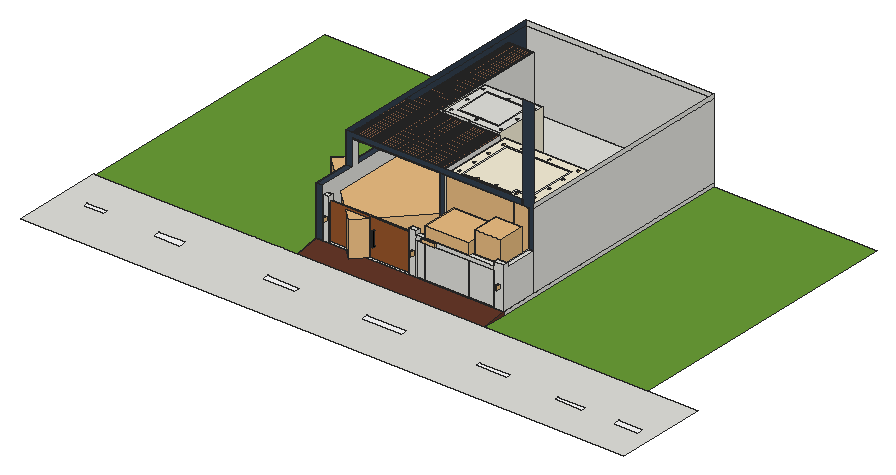
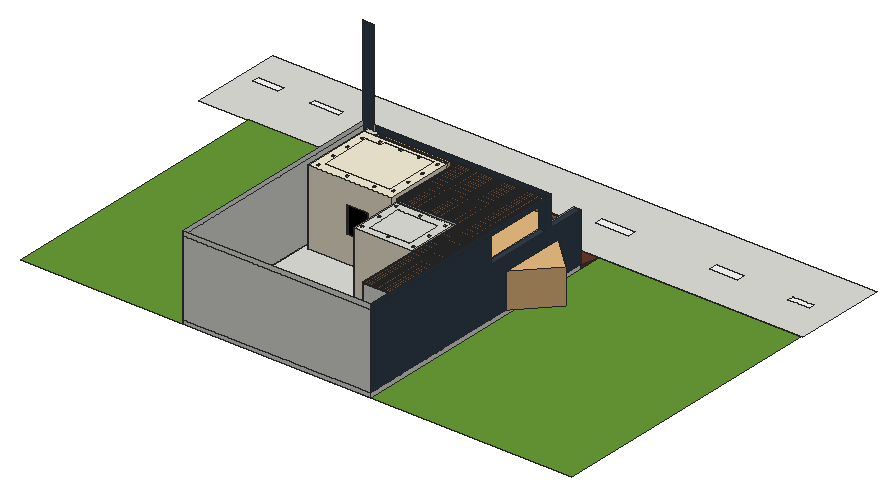
# SketchUp Ruby script. Lengths in inches.
U = 1.inch
M = Sketchup.active_model
def pt(a) = Geom::Point3d.new(a.map { |v| v * U })
def face(e, loops, mat)
  f = e.add_face(loops[0].map { |a| pt(a) })
  loops[1..].each { |l| e.add_face(l.map { |a| pt(a) }).erase! }
  f.material = f.back_material = mat if mat
  f
end
# faces: each face lists its corners as indices into pts; further lists are holes
def faces(e, pts, list, mat = nil) = list.each { |f| face(e, (f[0].is_a?(Array) ? f : [f]).map { |l| l.map { |i| pts[i] } }, mat) }
# xy, xz, yz: faces in a plane at the given z, y or x. An outline is a flat list of corners, or four numbers for a rectangle; further outlines are holes
def ring(l) = l.size == 4 ? [[l[0], l[1]], [l[2], l[1]], [l[2], l[3]], [l[0], l[3]]] : l.each_slice(2).to_a
def flat(e, list, mat, &to3) = list.each { |f| face(e, (f[0].is_a?(Array) ? f : [f]).map { |l| ring(l).map { |u, v| to3.(u, v) } }, mat) }
def xy(e, z, list, mat = nil) = flat(e, list, mat) { |x, y| [x, y, z] }
def xz(e, y, list, mat = nil) = flat(e, list, mat) { |x, z| [x, y, z] }
def yz(e, x, list, mat = nil) = flat(e, list, mat) { |y, z| [x, y, z] }
def lines(e, pts, list) = list.each { |a, b| e.add_line(pt(pts[a]), pt(pts[b])) }
# prism: a flat outline (further loops are holes) pulled along v
def prism(e, loops, v, mat = nil)
  f = face(e, loops, mat); d = Geom::Vector3d.new(v.map { |x| x * U })
  f.pushpull(f.normal.samedirection?(d) ? d.length : -d.length)
end
def box(e, o, s, mat = nil) = prism(e, [[o, [o[0] + s[0], o[1], o[2]], [o[0] + s[0], o[1] + s[1], o[2]], [o[0], o[1] + s[1], o[2]]]], [0, 0, s[2]], mat)
def at(x, y, z, deg = 0) = Geom::Transformation.translation(pt([x, y, z])) * Geom::Transformation.rotation(ORIGIN, Z_AXIS, deg.degrees)
def axes(o, x, y, z) = Geom::Transformation.new([*x, 0, *y, 0, *z, 0, *pt(o).to_a, 1])
def part(name) = M.definitions.add(name)
# library, detail: a bought-in or finely detailed component or shape, given as its bounding box
def library(name, o, s) = part(name).tap { |d| box(d.entities, o, s) }
def detail(e, o, s) = box(e.add_group.entities, o, s)
def put(e, d, t, mat = nil) = e.add_instance(d, t).tap { |i| i.material = mat if mat }
def group(e, t, mat = nil) = e.add_group.tap { |g| g.transformation = t; g.material = mat if mat }.entities
root = M.entities
M.materials.add("0400 AP 7301 PLUTO").color = [50, 63, 78]
M.materials.add("0897 AP 7835 CREAM CARESS").color = [247, 240, 216]
M.materials.add("Ceragres-Topcer-Brick-red-mat-6-4K").color = [99, 54, 40]
M.materials.add("Color_2").color = [255, 255, 255]
M.materials.add("Glass_Window_Neutral").color = [0, 0, 0]
M.materials["Glass_Window_Neutral"].alpha = 0.125
M.materials.add("Material60").color = [234, 198, 157]
M.materials.add("[Color M09]").color = [0, 0, 0]
M.materials.add("[Color M09]1").color = [0, 0, 0]
M.materials.add("[Grass Dark Green]").color = [106, 157, 55]
M.materials.add("[Wood Cherry Original]").color = [152, 86, 42]
M.materials.add("[Wood Veneer 02]").color = [190, 128, 91]
M.materials.add("ground1").color = [30, 21, 16]
M.materials.add("lz-doorbrown").color = [51, 28, 20]
M.materials.add("polished steel").color = [183, 187, 190]
M.materials.add("steel").color = [179, 179, 179]
c1 = part("Untitled")
xy(c1.entities,0,[[[158.81,26.5625,306.06,993.3125],[226.57,518.17,239.57,583.92],[225.28,357.51,237.28,411.51],[222.61,182.28,236.36,226.53],[239.71,931.55,251.46,972.3],[233.64,703.93,242.14,755.18],[240.05,835.03,248.8,880.53],[222.04,66.5,231.29,100.5]]])
xy(c1.entities,0,[[222.04,66.5,231.29,100.5],[222.61,182.28,236.36,226.53],[225.28,357.51,237.28,411.51],[226.57,518.17,239.57,583.92],[233.64,703.93,242.14,755.18],
  [240.05,835.03,248.8,880.53],[239.71,931.55,251.46,972.3]],"Color_2")
c2 = library("Senza",[-37.85,-41.61,-2.42],[41.39,41.83,53.67])
c3 = library("Cay chuoi",[-26.05,-21.66,0],[63.57,52.43,69.02])
c4 = library("шторы раздвинутые\#1",[23.6875,-79.1875,1.01],[68.3125,79.67,5.17])
c5 = library("door by lz",[5.91,-4.92,0],[35.43,6.61,78.74])
c6 = library("Спалня Венид",[0.07,-0.07,0],[84.71,86.8,39])
c7 = library("RANGE ROVER",[-63.71,-35.21,42.76],[182.88,182.88,64.08])
c8 = part("Bilal architect uae abu dhabi ")
put(c8.entities,c7,axes([104.22,-10.75,-48.75],[0.98727,0.57,0],[-0.57,0.98727,0],[0,0,1.14]),"Material60")
c9 = part("faewg")
xy(c9.entities,0,[[0,-3,2,0]])
xy(c9.entities,1,[[0,-2,2,0]])
xy(c9.entities,23,[[0,-2,2,0]])
xy(c9.entities,24,[[0,-3,2,0]])
xz(c9.entities,-3,[[0,0,2,24]],"polished steel")
xz(c9.entities,-2,[[0,1,2,23]])
xz(c9.entities,0,[[0,0,2,1],[0,23,2,24]])
yz(c9.entities,0,[[-3,0,-3,24,0,24,0,23,-2,23,-2,1,0,1,0,0]])
yz(c9.entities,2,[[-3,0,0,0,0,1,-2,1,-2,23,0,23,0,24,-3,24]])
c10 = part("reg")
xy(c10.entities,0,[[-8.95,3,59.93,5]],"[Wood Veneer 02]")
xy(c10.entities,18,[[51.93,0,53.93,3]],"[Wood Veneer 02]")
xy(c10.entities,19,[[51.93,1,53.93,3]],"[Color M09]")
xy(c10.entities,41,[[51.93,1,53.93,3]],"[Color M09]")
xy(c10.entities,42,[[51.93,0,53.93,3]],"[Color M09]")
xy(c10.entities,61,[[-8.95,3,59.93,5]],"[Wood Veneer 02]")
xz(c10.entities,0,[[51.93,18,53.93,42]],"[Color M09]")
xz(c10.entities,1,[[51.93,19,53.93,41]],"[Color M09]")
xz(c10.entities,3,[[[-8.95,0,59.93,61],[51.93,41,53.93,42],[51.93,18,53.93,19]]],"[Wood Cherry Original]")
xz(c10.entities,3,[[51.93,18,53.93,19],[51.93,41,53.93,42]],"[Wood Veneer 02]")
xz(c10.entities,5,[[-8.95,0,59.93,61]],"[Wood Veneer 02]")
yz(c10.entities,-8.95,[[3,0,5,61]],"[Wood Veneer 02]")
yz(c10.entities,51.93,[[0,18,0,42,3,42,3,41,1,41,1,19,3,19,3,18]],"[Color M09]")
yz(c10.entities,53.93,[[0,18,3,18,3,19,1,19,1,41,3,41,3,42,0,42]],"[Color M09]")
yz(c10.entities,59.93,[[3,0,5,61]],"[Wood Veneer 02]")
put(c10.entities,c9,axes([51.93,5.4375,42],[1,0,0],[0,-1,0],[0,0,-1]),"steel")
c11 = part("gbsrtn")
put(c11.entities,c10,at(402.95,-3,0))
put(c11.entities,c10,axes([522.82,-3,0],[-1,0,0],[0,1,0],[0,0,1]),"[Wood Veneer 02]")
c12 = library("Sliding windows",[297.42,-0.89,0.35],[194.88,8.85,122.84])
c13 = library("Group23\#1",[-12,-48,0],[24,96,0.39])
c14 = library("Wall Light 02",[0,0,0],[3.15,6.76,4.53])
c15 = library("JOHN_K",[0.08,0,0],[23.74,5.375,2])
c16 = part("Window")
xy(c16.entities,31.72,[[-0.78,88.6,2.72,128.1]])
xy(c16.entities,34.95,[[0.84,91.53,1.05,97.58],[1.05,91.53,1.42,106.59],[1.42,91.53,2.72,106.59],[0.84,97.58,1.05,98.18],[0.84,98.18,1.05,106.59]])
xy(c16.entities,34.95,[[-0.78,91.53,0.84,106.59]],"[Wood Cherry Original]")
xy(c16.entities,35.27,[[1.05,110.09,2.72,125.14]])
xy(c16.entities,35.27,[[-0.78,110.09,0.97,125.14]],"[Wood Cherry Original]")
xy(c16.entities,58.35,[[2.72,108.74,3.8,109.74]])
xy(c16.entities,77.8125,[[0.97,110.09,1.05,125.14]])
xy(c16.entities,77.8125,[[-0.78,110.09,2.72,125.14]],"[Wood Cherry Original]")
xy(c16.entities,77.93,[[1.05,91.53,1.42,106.59],[1.42,91.53,2.72,106.59]])
xy(c16.entities,77.93,[[-0.78,91.53,0.84,106.59]],"[Wood Cherry Original]")
xy(c16.entities,80.72,[[-0.78,88.6,2.72,128.1]])
xz(c16.entities,88.6,[[-0.78,31.72,2.72,80.72]])
xz(c16.entities,91.53,[[1.05,34.95,1.42,77.93],[1.42,34.95,2.72,77.93]])
xz(c16.entities,91.53,[[-0.78,34.95,0.84,77.93]],"[Wood Cherry Original]")
xz(c16.entities,106.59,[[0.84,34.95,1.05,77.93],[0.84,34.95,2.72,77.93]])
xz(c16.entities,106.59,[[-0.78,34.95,0.84,77.93]],"[Wood Cherry Original]")
xz(c16.entities,108.74,[[3.8,54.35,4.22,54.6,4.22,59.47,2.72,59.97,2.72,58.35,3.8,58.35]])
xz(c16.entities,109.74,[[3.8,54.35,3.8,58.35,2.72,58.35,2.72,59.97,4.22,59.47,4.22,54.6]])
xz(c16.entities,110.09,[[1.05,35.27,2.72,77.8125]])
xz(c16.entities,110.09,[[-0.78,35.27,0.97,77.8125]],"[Wood Cherry Original]")
xz(c16.entities,125.14,[[0.97,35.27,1.05,80.72],[1.05,35.27,2.72,77.8125]])
xz(c16.entities,125.14,[[-0.78,35.27,0.97,77.8125]],"[Wood Cherry Original]")
xz(c16.entities,128.1,[[-0.78,31.72,2.72,80.72]])
yz(c16.entities,-0.78,[[[88.6,31.72,128.1,80.72],[91.53,34.95,106.59,77.93],[110.09,35.27,125.14,77.8125]]],"[Wood Cherry Original]")
yz(c16.entities,1.05,[[91.53,34.95,106.59,77.93],[110.09,35.27,125.14,77.8125]],"Glass_Window_Neutral")
yz(c16.entities,1.42,[[91.53,34.95,106.59,77.93]])
yz(c16.entities,2.72,[[[88.6,31.72,108.35,80.72],[91.53,34.95,106.59,77.93]],[[108.35,31.72,128.1,80.72],[110.09,35.27,125.14,77.8125],[108.74,58.35,109.74,59.97]]])
yz(c16.entities,3.8,[[108.74,54.35,109.74,58.35]])
yz(c16.entities,4.22,[[108.74,54.6,109.74,59.47]])
p = [[4.22,108.74,54.6],[3.8,108.74,54.35],[3.8,109.74,54.35],[4.22,109.74,54.6],[2.72,109.74,59.97],[2.72,108.74,59.97],
  [4.22,108.74,59.47],[4.22,109.74,59.47],[-0.78,86.4,89.94],[-0.78,86.44,89.94],[15.22,130.69,89.94],[15.22,130.65,89.94],
  [-0.78,86.44,28.19],[-0.78,86.4,28.19],[7.72,130.69,89.94],[7.72,130.65,89.94]]
faces(c16.entities,p,[[0,1,2,3],[4,5,6,7]])
lines(c16.entities,p,[[8,9],[10,11],[12,13],[14,15]])
c17 = part("Group\#7")
xy(c17.entities,0,[[1.02,0,0.76,0.03,0.51,0.14,0.3,0.3,0.14,0.51,0.03,0.76,0,1.02,0.03,1.28,0.14,1.53,0.3,1.74,0.51,1.9,0.76,2.01,1.02,2.04,1.28,2.01,1.53,1.9,1.74,1.74,1.9,1.53,2.01,1.28,2.04,1.02,2.01,0.76,1.9,0.51,1.74,0.3,1.53,0.14,1.28,0.03]])
c18 = part("Group\#9")
detail(c18.entities,[3.14,3.14,12.38],[2.62,2.62,0.48])
put(c18.entities,c17,at(3.43,3.43,12.51))
c19 = part("Group450\#1")
box(c19.entities,[-75,-146,0],[1,110,0.375])
c20 = part("Group451\#1")
box(c20.entities,[-73.8125,-146,0],[1,110,0.375])
c21 = part("Group452\#1")
box(c21.entities,[-72.625,-146,0],[1,110,0.375])
c22 = part("Group453\#1")
box(c22.entities,[-71.4375,-146,0],[1,110,0.375])
c23 = part("Group454\#1")
box(c23.entities,[-70.25,-146,0],[1,110,0.375])
c24 = part("Group455\#1")
box(c24.entities,[-69.0625,-146,0],[1,110,0.375])
c25 = part("Group456\#1")
box(c25.entities,[-67.875,-146,0],[1,110,0.375])
c26 = part("Group457\#1")
box(c26.entities,[-66.6875,-146,0],[1,110,0.375])
c27 = part("Group458\#1")
xy(c27.entities,0,[[-65,-156,-65,-146,-65.5,-146,-65.5,-36,-65,-36,-65,156,-64.5,156,-64.5,-156]])
xy(c27.entities,0.375,[[-65,-156,-64.5,-156,-64.5,156,-65,156,-65,-36,-65.5,-36,-65.5,-146,-65,-146]])
yz(c27.entities,-65.5,[[-146,0,-36,0.375]])
yz(c27.entities,-64.5,[[-156,0,156,0.375]])
c28 = part("Group459\#1")
box(c28.entities,[-64.3125,-156,0],[1,312,0.375])
c29 = part("Group460\#1")
box(c29.entities,[-63.125,-156,0],[1,312,0.375])
c30 = part("Group461\#1")
box(c30.entities,[-61.9375,-156,0],[1,312,0.375])
c31 = part("Group462\#1")
box(c31.entities,[-60.75,-156,0],[1,312,0.375])
c32 = part("Group463\#1")
box(c32.entities,[-59.5625,-156,0],[1,312,0.375])
c33 = part("Group464\#1")
box(c33.entities,[-58.375,-156,0],[1,312,0.375])
c34 = part("Group465\#1")
box(c34.entities,[-57.1875,-156,0],[1,312,0.375])
c35 = part("Group466\#1")
box(c35.entities,[-56,-156,0],[1,312,0.375])
c36 = part("Group467\#1")
box(c36.entities,[-54.8125,-156,0],[1,312,0.375])
c37 = part("Group468\#1")
box(c37.entities,[-53.625,-156,0],[1,312,0.375])
c38 = part("Group469\#1")
box(c38.entities,[-52.4375,-156,0],[1,312,0.375])
c39 = part("Group470\#1")
box(c39.entities,[-51.25,-156,0],[1,312,0.375])
c40 = part("Group471\#1")
box(c40.entities,[-50.0625,-156,0],[1,312,0.375])
c41 = part("Group472\#1")
box(c41.entities,[-48.875,-156,0],[1,312,0.375])
c42 = part("Group473\#1")
box(c42.entities,[-47.6875,-156,0],[1,312,0.375])
c43 = part("Group474\#1")
box(c43.entities,[-46.5,-156,0],[1,312,0.375])
c44 = part("Group475\#1")
box(c44.entities,[-45.3125,-156,0],[1,312,0.375])
c45 = part("Group476\#1")
box(c45.entities,[-44.125,-156,0],[1,312,0.375])
c46 = part("Group477\#1")
box(c46.entities,[-42.9375,-156,0],[1,312,0.375])
c47 = part("Group478\#1")
box(c47.entities,[-41.75,-156,0],[1,312,0.375])
c48 = part("Group479\#1")
box(c48.entities,[-40.5625,-156,0],[1,312,0.375])
c49 = part("Group480\#1")
box(c49.entities,[-39.375,-156,0],[1,312,0.375])
c50 = part("Group481\#1")
box(c50.entities,[-38.1875,-156,0],[1,312,0.375])
c51 = part("Group482\#1")
box(c51.entities,[-37,-156,0],[1,312,0.375])
c52 = part("Group483\#1")
box(c52.entities,[-35.8125,-156,0],[1,312,0.375])
c53 = part("Group484\#1")
box(c53.entities,[-34.625,-156,0],[1,312,0.375])
c54 = part("Group485\#1")
box(c54.entities,[-33.4375,-156,0],[1,312,0.375])
c55 = part("Group486\#1")
box(c55.entities,[-32.25,-156,0],[1,312,0.375])
c56 = part("Group487\#1")
box(c56.entities,[-31.0625,-156,0],[1,312,0.375])
c57 = part("Group488\#1")
box(c57.entities,[-29.875,-156,0],[1,312,0.375])
c58 = part("Group489\#1")
box(c58.entities,[-28.6875,-156,0],[1,312,0.375])
c59 = part("Group490\#1")
box(c59.entities,[-27.5,-156,0],[1,312,0.375])
c60 = part("Group491\#1")
box(c60.entities,[-26.3125,-156,0],[1,312,0.375])
c61 = part("Group492\#1")
xy(c61.entities,0,[[-25.125,-156,-25.125,156,-24.3125,156,-24.3125,-36,-24.125,-36,-24.125,-156]])
xy(c61.entities,0.375,[[-25.125,-156,-24.125,-156,-24.125,-36,-24.3125,-36,-24.3125,156,-25.125,156]])
xz(c61.entities,-156,[[-25.125,0,-24.125,0.375]])
yz(c61.entities,-25.125,[[-156,0,156,0.375]])
yz(c61.entities,-24.125,[[-156,0,-36,0.375]])
c62 = part("Group493\#1")
box(c62.entities,[-23.9375,-156,0],[1,120,0.375])
c63 = part("Group494\#1")
box(c63.entities,[-22.75,-156,0],[1,120,0.375])
c64 = part("Group495\#1")
box(c64.entities,[-21.5625,-156,0],[1,120,0.375])
c65 = part("Group496\#1")
box(c65.entities,[-20.375,-156,0],[1,120,0.375])
c66 = part("Group497\#1")
box(c66.entities,[-19.1875,-156,0],[1,120,0.375])
c67 = part("Group498\#1")
box(c67.entities,[-18,-156,0],[1,120,0.375])
c68 = part("Group499\#1")
box(c68.entities,[-16.8125,-156,0],[1,120,0.375])
c69 = part("Group500\#1")
box(c69.entities,[-15.625,-156,0],[1,120,0.375])
c70 = part("Group501\#1")
box(c70.entities,[-14.4375,-156,0],[1,120,0.375])
c71 = part("Group502\#1")
box(c71.entities,[-13.25,-156,0],[1,120,0.375])
c72 = part("Group503\#1")
box(c72.entities,[-12.0625,-156,0],[1,120,0.375])
c73 = part("Group504\#1")
box(c73.entities,[-10.875,-156,0],[1,120,0.375])
c74 = part("Group505\#1")
box(c74.entities,[-9.6875,-156,0],[1,120,0.375])
c75 = part("Group506\#1")
box(c75.entities,[-8.5,-156,0],[1,120,0.375])
c76 = part("Group507\#1")
box(c76.entities,[-7.3125,-156,0],[1,120,0.375])
c77 = part("Group508\#1")
box(c77.entities,[-6.125,-156,0],[1,120,0.375])
c78 = part("Group509\#1")
box(c78.entities,[-4.9375,-156,0],[1,120,0.375])
c79 = part("Group510\#1")
box(c79.entities,[-3.75,-156,0],[1,120,0.375])
c80 = part("Group511\#1")
box(c80.entities,[-2.5625,-156,0],[1,120,0.375])
c81 = part("Group512\#1")
box(c81.entities,[-1.375,-156,0],[1,120,0.375])
c82 = part("Group513\#1")
box(c82.entities,[-0.1875,-156,0],[1,120,0.375])
c83 = part("Group514\#1")
box(c83.entities,[1,-156,0],[1,120,0.375])
c84 = part("Group515\#1")
box(c84.entities,[2.1875,-156,0],[1,120,0.375])
c85 = part("Group516\#1")
box(c85.entities,[3.375,-156,0],[1,120,0.375])
c86 = part("Group517\#1")
box(c86.entities,[4.5625,-156,0],[1,120,0.375])
c87 = part("Group518\#1")
box(c87.entities,[5.75,-156,0],[1,120,0.375])
c88 = part("Group519\#1")
box(c88.entities,[6.9375,-156,0],[1,120,0.375])
c89 = part("Group520\#1")
box(c89.entities,[8.125,-156,0],[1,120,0.375])
c90 = part("Group521\#1")
box(c90.entities,[9.3125,-156,0],[1,120,0.375])
c91 = part("Group522\#1")
box(c91.entities,[10.5,-156,0],[1,120,0.375])
c92 = part("Group523\#1")
box(c92.entities,[11.6875,-156,0],[1,120,0.375])
c93 = part("Group524\#1")
box(c93.entities,[12.875,-156,0],[1,120,0.375])
c94 = part("Group525\#1")
box(c94.entities,[14.0625,-156,0],[1,120,0.375])
c95 = part("Group526\#1")
box(c95.entities,[15.25,-156,0],[1,120,0.375])
c96 = part("Group527\#1")
box(c96.entities,[16.4375,-156,0],[1,120,0.375])
c97 = part("Group528\#1")
box(c97.entities,[17.625,-156,0],[1,120,0.375])
c98 = part("Group529\#1")
box(c98.entities,[18.8125,-156,0],[1,120,0.375])
c99 = part("Group530\#1")
box(c99.entities,[20,-156,0],[1,120,0.375])
c100 = part("Group531\#1")
box(c100.entities,[21.1875,-156,0],[1,120,0.375])
c101 = part("Group532\#1")
box(c101.entities,[22.375,-156,0],[1,120,0.375])
c102 = part("Group533\#1")
box(c102.entities,[23.5625,-156,0],[1,120,0.375])
c103 = part("Group534\#1")
box(c103.entities,[24.75,-156,0],[1,120,0.375])
c104 = part("Group535\#1")
box(c104.entities,[25.9375,-156,0],[1,120,0.375])
c105 = part("Group536\#1")
box(c105.entities,[27.125,-156,0],[1,120,0.375])
c106 = part("Group537\#1")
box(c106.entities,[28.3125,-156,0],[1,120,0.375])
c107 = part("Group538\#1")
box(c107.entities,[29.5,-156,0],[1,120,0.375])
c108 = part("Group539\#1")
box(c108.entities,[30.6875,-156,0],[1,120,0.375])
c109 = part("Group540\#1")
box(c109.entities,[31.875,-156,0],[1,120,0.375])
c110 = part("Group541\#1")
box(c110.entities,[33.0625,-156,0],[1,120,0.375])
c111 = part("Group542\#1")
box(c111.entities,[34.25,-156,0],[1,120,0.375])
c112 = part("Group543\#1")
box(c112.entities,[35.4375,-156,0],[1,120,0.375])
c113 = part("Group544\#1")
box(c113.entities,[36.625,-156,0],[1,120,0.375])
c114 = part("Group545\#1")
box(c114.entities,[37.8125,-156,0],[1,120,0.375])
c115 = part("Group546\#1")
box(c115.entities,[39,-156,0],[1,120,0.375])
c116 = part("Group547\#1")
box(c116.entities,[40.1875,-156,0],[1,120,0.375])
c117 = part("Group548\#1")
box(c117.entities,[41.375,-156,0],[1,120,0.375])
c118 = part("Group549\#1")
box(c118.entities,[42.5625,-156,0],[1,120,0.375])
c119 = part("Group550\#1")
box(c119.entities,[43.75,-156,0],[1,120,0.375])
c120 = part("Group551\#1")
box(c120.entities,[44.9375,-156,0],[1,120,0.375])
c121 = part("Group552\#1")
box(c121.entities,[46.125,-156,0],[1,120,0.375])
c122 = part("Group553\#1")
box(c122.entities,[47.3125,-156,0],[1,120,0.375])
c123 = part("Group554\#1")
box(c123.entities,[48.5,-156,0],[1,120,0.375])
c124 = part("Group555\#1")
box(c124.entities,[49.6875,-156,0],[1,120,0.375])
c125 = part("Group556\#1")
box(c125.entities,[50.875,-156,0],[1,120,0.375])
c126 = part("Group557\#1")
box(c126.entities,[52.0625,-156,0],[1,120,0.375])
c127 = part("Group558\#1")
box(c127.entities,[53.25,-156,0],[1,120,0.375])
c128 = part("Group559\#1")
box(c128.entities,[54.4375,-156,0],[1,120,0.375])
c129 = part("Group560\#1")
box(c129.entities,[55.625,-156,0],[1,120,0.375])
c130 = part("Group561\#1")
box(c130.entities,[56.8125,-156,0],[1,120,0.375])
c131 = part("Group562\#1")
box(c131.entities,[58,-156,0],[1,120,0.375])
c132 = part("Group563\#1")
box(c132.entities,[59.1875,-156,0],[1,120,0.375])
c133 = part("Group564\#1")
box(c133.entities,[60.375,-156,0],[1,120,0.375])
c134 = part("Group565\#1")
box(c134.entities,[61.5625,-156,0],[1,120,0.375])
c135 = part("Group566\#1")
box(c135.entities,[62.75,-156,0],[1,120,0.375])
c136 = part("Group567\#1")
box(c136.entities,[63.9375,-156,0],[1,120,0.375])
c137 = part("Group568\#1")
box(c137.entities,[65.125,-156,0],[1,120,0.375])
c138 = part("Group569\#1")
box(c138.entities,[66.3125,-156,0],[1,120,0.375])
c139 = part("Group570\#1")
box(c139.entities,[67.5,-156,0],[1,120,0.375])
c140 = part("Group571\#1")
box(c140.entities,[68.6875,-156,0],[1,120,0.375])
c141 = part("Group572\#1")
box(c141.entities,[69.875,-156,0],[1,120,0.375])
c142 = part("Group573\#1")
box(c142.entities,[71.0625,-156,0],[1,120,0.375])
c143 = part("Group574\#1")
box(c143.entities,[72.25,-156,0],[1,120,0.375])
c144 = part("Group575\#1")
box(c144.entities,[73.4375,-156,0],[1,120,0.375])
c145 = part("Group576\#1")
xy(c145.entities,0,[[74.625,-156,75,-36]])
xy(c145.entities,0.375,[[74.625,-156,75,-36]])
yz(c145.entities,74.625,[[-156,0,-36,0.375]])
c146 = part("Group448\#1")
put(c146.entities,c19,at(0,0,0))
put(c146.entities,c20,at(0,0,0))
put(c146.entities,c21,at(0,0,0))
put(c146.entities,c22,at(0,0,0))
put(c146.entities,c23,at(0,0,0))
put(c146.entities,c24,at(0,0,0))
put(c146.entities,c25,at(0,0,0))
put(c146.entities,c26,at(0,0,0))
put(c146.entities,c27,at(0,0,0))
put(c146.entities,c28,at(0,0,0))
put(c146.entities,c29,at(0,0,0))
put(c146.entities,c30,at(0,0,0))
put(c146.entities,c31,at(0,0,0))
put(c146.entities,c32,at(0,0,0))
put(c146.entities,c33,at(0,0,0))
put(c146.entities,c34,at(0,0,0))
put(c146.entities,c35,at(0,0,0))
put(c146.entities,c36,at(0,0,0))
put(c146.entities,c37,at(0,0,0))
put(c146.entities,c38,at(0,0,0))
put(c146.entities,c39,at(0,0,0))
put(c146.entities,c40,at(0,0,0))
put(c146.entities,c41,at(0,0,0))
put(c146.entities,c42,at(0,0,0))
put(c146.entities,c43,at(0,0,0))
put(c146.entities,c44,at(0,0,0))
put(c146.entities,c45,at(0,0,0))
put(c146.entities,c46,at(0,0,0))
put(c146.entities,c47,at(0,0,0))
put(c146.entities,c48,at(0,0,0))
put(c146.entities,c49,at(0,0,0))
put(c146.entities,c50,at(0,0,0))
put(c146.entities,c51,at(0,0,0))
put(c146.entities,c52,at(0,0,0))
put(c146.entities,c53,at(0,0,0))
put(c146.entities,c54,at(0,0,0))
put(c146.entities,c55,at(0,0,0))
put(c146.entities,c56,at(0,0,0))
put(c146.entities,c57,at(0,0,0))
put(c146.entities,c58,at(0,0,0))
put(c146.entities,c59,at(0,0,0))
put(c146.entities,c60,at(0,0,0))
put(c146.entities,c61,at(0,0,0))
put(c146.entities,c62,at(0,0,0))
put(c146.entities,c63,at(0,0,0))
put(c146.entities,c64,at(0,0,0))
put(c146.entities,c65,at(0,0,0))
put(c146.entities,c66,at(0,0,0))
put(c146.entities,c67,at(0,0,0))
put(c146.entities,c68,at(0,0,0))
put(c146.entities,c69,at(0,0,0))
put(c146.entities,c70,at(0,0,0))
put(c146.entities,c71,at(0,0,0))
put(c146.entities,c72,at(0,0,0))
put(c146.entities,c73,at(0,0,0))
put(c146.entities,c74,at(0,0,0))
put(c146.entities,c75,at(0,0,0))
put(c146.entities,c76,at(0,0,0))
put(c146.entities,c77,at(0,0,0))
put(c146.entities,c78,at(0,0,0))
put(c146.entities,c79,at(0,0,0))
put(c146.entities,c80,at(0,0,0))
put(c146.entities,c81,at(0,0,0))
put(c146.entities,c82,at(0,0,0))
put(c146.entities,c83,at(0,0,0))
put(c146.entities,c84,at(0,0,0))
put(c146.entities,c85,at(0,0,0))
put(c146.entities,c86,at(0,0,0))
put(c146.entities,c87,at(0,0,0))
put(c146.entities,c88,at(0,0,0))
put(c146.entities,c89,at(0,0,0))
put(c146.entities,c90,at(0,0,0))
put(c146.entities,c91,at(0,0,0))
put(c146.entities,c92,at(0,0,0))
put(c146.entities,c93,at(0,0,0))
put(c146.entities,c94,at(0,0,0))
put(c146.entities,c95,at(0,0,0))
put(c146.entities,c96,at(0,0,0))
put(c146.entities,c97,at(0,0,0))
put(c146.entities,c98,at(0,0,0))
put(c146.entities,c99,at(0,0,0))
put(c146.entities,c100,at(0,0,0))
put(c146.entities,c101,at(0,0,0))
put(c146.entities,c102,at(0,0,0))
put(c146.entities,c103,at(0,0,0))
put(c146.entities,c104,at(0,0,0))
put(c146.entities,c105,at(0,0,0))
put(c146.entities,c106,at(0,0,0))
put(c146.entities,c107,at(0,0,0))
put(c146.entities,c108,at(0,0,0))
put(c146.entities,c109,at(0,0,0))
put(c146.entities,c110,at(0,0,0))
put(c146.entities,c111,at(0,0,0))
put(c146.entities,c112,at(0,0,0))
put(c146.entities,c113,at(0,0,0))
put(c146.entities,c114,at(0,0,0))
put(c146.entities,c115,at(0,0,0))
put(c146.entities,c116,at(0,0,0))
put(c146.entities,c117,at(0,0,0))
put(c146.entities,c118,at(0,0,0))
put(c146.entities,c119,at(0,0,0))
put(c146.entities,c120,at(0,0,0))
put(c146.entities,c121,at(0,0,0))
put(c146.entities,c122,at(0,0,0))
put(c146.entities,c123,at(0,0,0))
put(c146.entities,c124,at(0,0,0))
put(c146.entities,c125,at(0,0,0))
put(c146.entities,c126,at(0,0,0))
put(c146.entities,c127,at(0,0,0))
put(c146.entities,c128,at(0,0,0))
put(c146.entities,c129,at(0,0,0))
put(c146.entities,c130,at(0,0,0))
put(c146.entities,c131,at(0,0,0))
put(c146.entities,c132,at(0,0,0))
put(c146.entities,c133,at(0,0,0))
put(c146.entities,c134,at(0,0,0))
put(c146.entities,c135,at(0,0,0))
put(c146.entities,c136,at(0,0,0))
put(c146.entities,c137,at(0,0,0))
put(c146.entities,c138,at(0,0,0))
put(c146.entities,c139,at(0,0,0))
put(c146.entities,c140,at(0,0,0))
put(c146.entities,c141,at(0,0,0))
put(c146.entities,c142,at(0,0,0))
put(c146.entities,c143,at(0,0,0))
put(c146.entities,c144,at(0,0,0))
put(c146.entities,c145,at(0,0,0))
xy(root,0,[[625.96,147.25,886.89,604.875],[3.02,147.3125,325.96,604.875]],"[Grass Dark Green]")
xy(root,6,[[[325.96,184.875,325.96,604.875,625.96,604.875,625.96,244.875,475.96,244.875,475.96,364.875,471.96,364.875,471.96,455.625,379.83,455.625,379.83,370.875,422.96,370.875,422.96,364.875,376.64,364.875,376.64,556.875,335.96,556.875,335.96,184.875],[483.96,252.875,617.96,364.875]]])
xy(root,30,[[483.96,244.875,593.96,252.875],[593.96,244.875,617.96,252.875]])
xy(root,66,[[379.83,364.875,420.77,371.625]])
xy(root,84.9375,[[325.96,184.875,335.96,244.875],[325.96,254.875,335.96,364.875]],"0400 AP 7301 PLUTO")
xy(root,102,[[379.83,364.875,381.96,370.875],[381.96,364.875,420.77,370.875],[422.96,364.875,471.96,370.875],[379.83,370.875,381.96,371.625],[381.96,370.875,420.77,371.625]])
xy(root,126,[[593.96,244.875,593.96,252.875,617.96,252.875,617.96,244.875,608.46,244.875,608.46,245.875,607.46,245.875,607.46,244.875],[[420.77,370.875,420.77,371.625,379.83,371.625,379.83,455.625,471.96,455.625,471.96,370.875],[433.73,383.84,458.99,383.84,458.99,442.66,392.79,442.66,392.79,384.59,433.73,384.59]],[434.73,384.84,434.73,385.59,393.79,385.59,393.79,441.66,457.99,441.66,457.99,384.84]])
xy(root,126,[[[483.96,244.875,483.96,364.875,617.96,364.875,617.96,252.875,593.96,252.875,593.96,244.875],[498.96,259.875,578.96,259.875,578.96,267.875,602.96,267.875,602.96,349.875,498.96,349.875]],[499.96,260.875,499.96,348.875,601.96,348.875,601.96,268.875,577.96,268.875,577.96,260.875]],"0897 AP 7835 CREAM CARESS")
xz(root,184.875,[[325.96,6,335.96,84.9375]],"0400 AP 7301 PLUTO")
xz(root,244.875,[[475.96,6,625.96,6,625.96,278,608.46,278,608.46,126,617.96,126,617.96,30,483.96,30,483.96,126,475.96,126],[325.96,84.9375,335.96,84.9375,335.96,126,607.46,126,607.46,134,325.96,134]],"0400 AP 7301 PLUTO")
xz(root,252.875,[[483.96,6,617.96,30],[593.96,30,617.96,126]])
xz(root,254.875,[[325.96,84.9375,335.96,126]],"0400 AP 7301 PLUTO")
xz(root,364.875,[[376.64,6,422.96,6,422.96,102,420.77,102,420.77,66,379.83,66,379.83,102,471.96,102,471.96,6,475.96,6,475.96,126,376.64,126]])
xz(root,364.875,[[325.96,84.9375,335.96,126]],"0400 AP 7301 PLUTO")
xz(root,364.875,[[483.96,6,617.96,126]],"0897 AP 7835 CREAM CARESS")
xz(root,370.875,[[420.77,102,422.96,126],[422.96,102,471.96,126]])
xz(root,371.625,[[379.83,102,381.96,126],[381.96,102,420.77,126]])
xz(root,455.625,[[379.83,6,471.96,126]],"0897 AP 7835 CREAM CARESS")
xz(root,556.875,[[335.96,6,376.64,126]])
xz(root,604.875,[[325.96,6,625.96,126],[325.96,126,625.96,134]])
yz(root,325.96,[[184.875,6,184.875,84.9375,244.875,84.9375,244.875,126,254.875,126,254.875,84.9375,364.875,84.9375,364.875,126,604.875,126,604.875,6],[244.875,126,604.875,134]],"0400 AP 7301 PLUTO")
yz(root,335.96,[[184.875,6,556.875,6,556.875,126,364.875,126,364.875,84.9375,254.875,84.9375,254.875,126,244.875,126,244.875,84.9375,184.875,84.9375]])
yz(root,376.64,[[364.875,6,556.875,126]])
yz(root,379.83,[[364.875,66,370.875,102],[370.875,66,371.625,102]])
yz(root,379.83,[[370.875,6,455.625,6,455.625,126,371.625,126,371.625,66,370.875,66]],"0897 AP 7835 CREAM CARESS")
yz(root,420.77,[[364.875,66,371.625,102],[370.875,102,371.625,126]])
yz(root,422.96,[[364.875,6,370.875,102]])
yz(root,471.96,[[364.875,6,364.875,102,370.875,102,370.875,126,455.625,126,455.625,6]],"0897 AP 7835 CREAM CARESS")
yz(root,475.96,[[244.875,6,364.875,126]])
yz(root,483.96,[[252.875,6,364.875,6,364.875,126,244.875,126,244.875,30,252.875,30]],"0897 AP 7835 CREAM CARESS")
yz(root,593.96,[[244.875,30,252.875,126]])
yz(root,607.46,[[244.875,126,245.875,134]])
yz(root,608.46,[[244.875,126,245.875,134]])
yz(root,617.96,[[244.875,30,252.875,126]])
yz(root,617.96,[[252.875,6,364.875,126]],"0897 AP 7835 CREAM CARESS")
yz(root,625.96,[[244.875,6,604.875,126],[244.875,126,604.875,134]])
put(root,c1,at(-26.5625,306.06,0,-90))
g1 = group(root,at(325.96,184.875,0))
xy(g1,0,[[0,-37.625,300,0],[0,0,300,420]])
xy(g1,6,[[[0,0,300,420],[150,8,292.05,60]]])
xy(g1,6,[[150,8,292.05,60]],"[Grass Dark Green]")
xz(g1,0,[[0,0,300,6]])
xz(g1,420,[[0,0,300,6]])
yz(g1,0,[[0,0,420,6]])
yz(g1,0,[[-37.625,0,0,6,0,0]],"Ceragres-Topcer-Brick-red-mat-6-4K")
yz(g1,300,[[0,0,420,6]])
yz(g1,300,[[-37.625,0,0,0,0,6]],"Ceragres-Topcer-Brick-red-mat-6-4K")
p = [[0,0,6],[0,-37.625,0],[300,-37.625,0],[300,0,6]]
faces(g1,p,[[0,1,2,3]],"Ceragres-Topcer-Brick-red-mat-6-4K")
put(root,c2,axes([607.87,238.875,8.99],[1,0,0],[0,1,0],[0,0,1.74588]))
put(root,c3,axes([527.0625,211.52,6],[1.11,0,0],[0,1.11,0],[0,0,1.11]),"ground1")
put(root,c4,axes([443.8,255.04,125.28],[1.6952,0,0],[0,0,1.50632],[0,-1,0]))
put(root,c5,axes([414.78,368.91,6],[1.38289,0,0],[0,1,0],[0,0,1.2192]),"lz-doorbrown")
put(root,c6,at(572.37,272.91,6,90))
g2 = group(root,at(618,184.875,6))
box(g2,[-282.05,0,0],[10,8,66])
xy(g2,0,[[-144.05,0,-144.05,8,0,8,0,60,7.95,60,7.95,0,-8,0,-8,2,-131.98,2,-131.98,0]])
xy(g2,54,[[-131.98,0,-8,2]])
xy(g2,60,[[-131.98,0,-8,8],[0,8,7.95,60]])
xy(g2,66,[[-144.05,0,-131.98,8],[-8,0,7.95,8]])
xz(g2,0,[[-144.05,0,-131.98,66],[-8,0,7.95,66],[-131.98,54,-8,60]])
xz(g2,2,[[-131.98,0,-8,54]])
xz(g2,8,[[-144.05,0,-144.05,66,-131.98,66,-131.98,60,-8,60,-8,66,0,66,0,0],[0,60,7.95,66]])
xz(g2,60,[[0,0,7.95,60]])
yz(g2,-144.05,[[0,0,8,66]])
yz(g2,-131.98,[[0,0,2,54],[0,60,8,66]])
yz(g2,-8,[[0,0,2,54],[0,60,8,66]])
yz(g2,0,[[8,0,60,60]])
yz(g2,7.95,[[0,0,60,0,60,60,8,60,8,66,0,66]])
put(root,c8,axes([324.89,218.58,6],[0.17714,0.74935,0],[0.74935,-0.17714,0],[0,0,0.77]))
put(root,c11,axes([-20.11,187.875,6.88],[0.92909,0,0],[0,1,0],[0,0,0.96914]),"[Wood Veneer 02]")
put(root,c12,axes([316.08,246.94,29.73],[0.56444,0,0],[0,0.54,0],[0,0,0.78154]))
put(root,c13,axes([605.96,244.875,78],[1,0,0],[0,0,1],[0,-1,0]),"[Wood Cherry Original]")
put(root,c14,axes([616.4,184.875,35.62],[1,0,0],[0,0,1],[0,-1,0]))
put(root,c14,axes([478.41,184.875,35.62],[1,0,0],[0,0,1],[0,-1,0]))
put(root,c14,axes([339.38,184.875,35.62],[1,0,0],[0,0,1],[0,-1,0]))
g3 = group(root,at(522.48,364.09,48.24),"[Color M09]")
xy(g3,0,[[0,0,33.48,0.79]])
xy(g3,1,[[0.93,0,32.55,0.39]])
xy(g3,40.76,[[0.93,0,32.55,0.39]])
xy(g3,41.76,[[0,0,33.48,0.79]])
xz(g3,0,[[[0,0,33.48,41.76],[0.93,1,32.55,40.76]]])
xz(g3,0.39,[[0.93,1,32.55,40.76]])
xz(g3,0.79,[[0,0,33.48,41.76]])
yz(g3,0,[[0,0,0.79,41.76]])
yz(g3,0.93,[[0,1,0.39,40.76]])
yz(g3,32.55,[[0,1,0.39,40.76]])
yz(g3,33.48,[[0,0,0.79,41.76]])
put(root,c15,axes([494.25,184.875,60],[1,0,0],[0,0,1],[0,-1,0]),"[Color M09]1")
put(root,c16,axes([512,367.625,42.79],[0,1.04,0],[-1.03072,0,0],[0,0,0.73326]))
put(root,c14,axes([603.82,244.48,77.82],[1,0,0],[0,0,1],[0,-1,0]))
put(root,c18,at(461.73,440.85,112.99))
put(root,c18,at(421.25,440.85,112.99))
put(root,c18,at(380.77,440.85,112.99))
put(root,c18,at(461.73,407.53,112.99))
put(root,c18,at(461.73,374.22,112.99))
put(root,c18,at(382.11,407.53,112.99))
put(root,c18,at(382.11,374.91,112.99))
put(root,c18,at(422.61,374.91,112.99))
put(root,c18,at(455.17,344.4,112.99))
put(root,c18,at(418.67,344.4,112.99))
put(root,c18,at(387.86,344.4,112.99))
put(root,c18,at(455.17,299.97,112.99))
put(root,c18,at(418.67,299.97,112.99))
put(root,c18,at(387.86,299.97,112.99))
put(root,c18,at(455.17,260.28,112.99))
put(root,c18,at(387.86,260.28,112.99))
put(root,c18,at(351.42,299.97,112.99))
put(root,c18,at(351.42,260.28,112.99))
put(root,c18,at(351.42,344.4,112.99))
put(root,c18,at(351.42,380.4,112.99))
put(root,c18,at(351.42,416.4,112.99))
put(root,c18,at(351.42,452.4,112.99))
put(root,c18,at(351.42,488.4,112.99))
put(root,c18,at(351.42,524.4,112.99))
put(root,c18,at(514.43,352.03,112.99))
put(root,c18,at(558.06,352.03,112.99))
put(root,c18,at(603.37,352.03,112.99))
put(root,c18,at(603.37,323.03,112.99))
put(root,c18,at(603.37,294.03,112.99))
put(root,c18,at(603.37,265.03,112.99))
put(root,c18,at(488.28,346.09,113.14))
put(root,c18,at(488.28,317.09,113.14))
put(root,c18,at(488.28,288.09,113.14))
put(root,c18,at(488.28,259.09,113.14))
put(root,c18,at(517.28,259.09,113.14))
put(root,c18,at(546.28,259.09,113.14))
put(root,c18,at(579.72,259.09,113.14))
g4 = group(root,at(392.79,383.84,126))
xy(g4,0,[[[40.9375,0,40.9375,0.75,0,0.75,0,58.82,66.2,58.82,66.2,0],[41.9375,1,65.2,1,65.2,57.82,1,57.82,1,1.75,41.9375,1.75]]])
g5 = group(root,at(607.46,245.875,126),"0400 AP 7301 PLUTO")
xz(g5,0,[[0,0,1,152]])
put(root,c146,at(400.96,400.875,126),"[Wood Veneer 02]")
g6 = group(root,at(498.96,259.875,126))
xy(g6,0,[[[0,0,0,90,104,90,104,8,80,8,80,0],[1,1,79,1,79,9,103,9,103,89,1,89]]])
